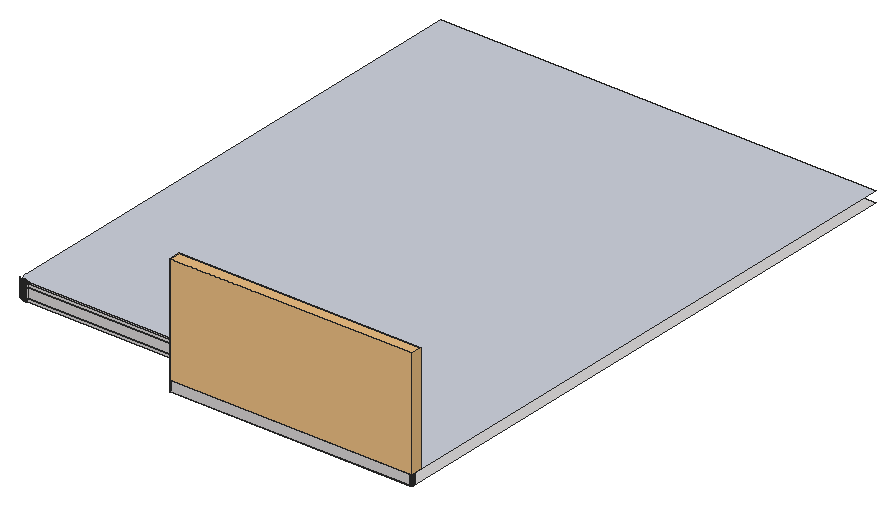
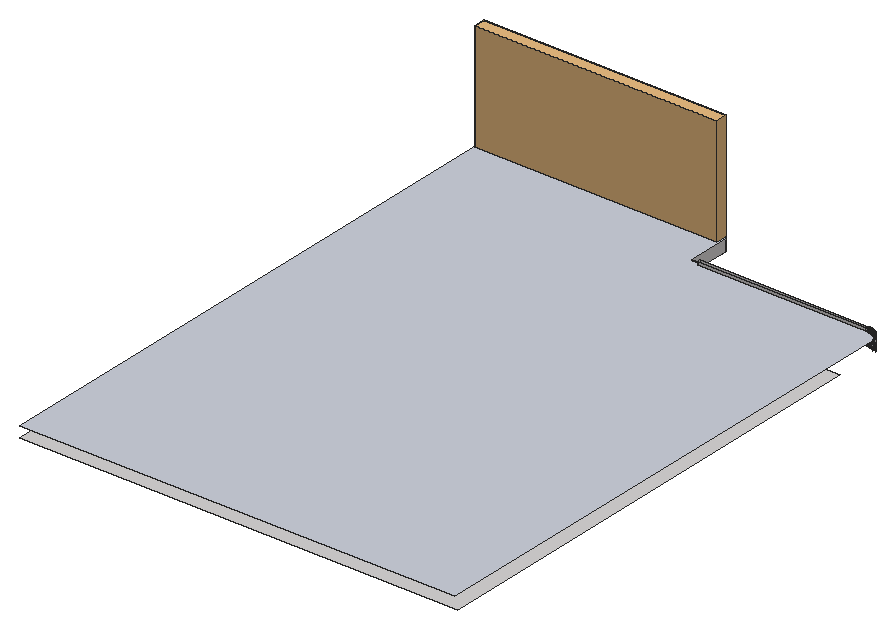
# SketchUp Ruby script. Lengths in inches.
U = 1.inch
M = Sketchup.active_model
def pt(a) = Geom::Point3d.new(a.map { |v| v * U })
def face(e, loops, mat)
  f = e.add_face(loops[0].map { |a| pt(a) })
  loops[1..].each { |l| e.add_face(l.map { |a| pt(a) }).erase! }
  f.material = f.back_material = mat if mat
  f
end
# faces: each face lists its corners as indices into pts; further lists are holes
def faces(e, pts, list, mat = nil) = list.each { |f| face(e, (f[0].is_a?(Array) ? f : [f]).map { |l| l.map { |i| pts[i] } }, mat) }
# xy, xz, yz: faces in a plane at the given z, y or x. An outline is a flat list of corners, or four numbers for a rectangle; further outlines are holes
def ring(l) = l.size == 4 ? [[l[0], l[1]], [l[2], l[1]], [l[2], l[3]], [l[0], l[3]]] : l.each_slice(2).to_a
def flat(e, list, mat, &to3) = list.each { |f| face(e, (f[0].is_a?(Array) ? f : [f]).map { |l| ring(l).map { |u, v| to3.(u, v) } }, mat) }
def xy(e, z, list, mat = nil) = flat(e, list, mat) { |x, y| [x, y, z] }
def xz(e, y, list, mat = nil) = flat(e, list, mat) { |x, z| [x, y, z] }
def yz(e, x, list, mat = nil) = flat(e, list, mat) { |y, z| [x, y, z] }
def lines(e, pts, list) = list.each { |a, b| e.add_line(pt(pts[a]), pt(pts[b])) }
# prism: a flat outline (further loops are holes) pulled along v
def prism(e, loops, v, mat = nil)
  f = face(e, loops, mat); d = Geom::Vector3d.new(v.map { |x| x * U })
  f.pushpull(f.normal.samedirection?(d) ? d.length : -d.length)
end
def box(e, o, s, mat = nil) = prism(e, [[o, [o[0] + s[0], o[1], o[2]], [o[0] + s[0], o[1] + s[1], o[2]], [o[0], o[1] + s[1], o[2]]]], [0, 0, s[2]], mat)
def at(x, y, z, deg = 0) = Geom::Transformation.translation(pt([x, y, z])) * Geom::Transformation.rotation(ORIGIN, Z_AXIS, deg.degrees)
def axes(o, x, y, z) = Geom::Transformation.new([*x, 0, *y, 0, *z, 0, *pt(o).to_a, 1])
def part(name) = M.definitions.add(name)
# library, detail: a bought-in or finely detailed component or shape, given as its bounding box
def library(name, o, s) = part(name).tap { |d| box(d.entities, o, s) }
def detail(e, o, s) = box(e.add_group.entities, o, s)
def put(e, d, t, mat = nil) = e.add_instance(d, t).tap { |i| i.material = mat if mat }
def group(e, t, mat = nil) = e.add_group.tap { |g| g.transformation = t; g.material = mat if mat }.entities
root = M.entities
M.materials.add("[Marble Carrara Floor Tile]").color = [204, 208, 219]
M.materials.add("[Quartz Light Brown]").color = [215, 212, 212]
c1 = library("Garniza_zaclona",[1.52,0,0],[127.96,8.15,78.72])
xy(root,246,[[215.88,155,215.76,155.01,215.65,155.02,215.41,155.06,215.3,155.08,215.1875,155.11,215.07,155.15,214.96,155.1875,214.85,155.23,214.74,155.28,214.64,155.33,214.53,155.38,214.43,155.44,214.33,155.51,214.24,155.57,214.14,155.64,213.96,155.8,213.8,155.96,213.64,156.14,213.57,156.24,213.51,156.33,213.44,156.43,213.38,156.53,213.33,156.64,213.28,156.74,213.23,156.85,213.15,157.07,213.11,157.1875,213.08,157.3,213.06,157.42,213.04,157.53,213.02,157.65,213.01,157.76,213,157.88,213,205,204,205,204,266,0,266,0,794,483,794,483,157.88,482.99,157.76,482.98,157.65,482.96,157.53,482.94,157.42,482.92,157.3,482.89,157.1875,482.85,157.07,482.8125,156.96,482.77,156.85,482.72,156.74,482.67,156.64,482.62,156.53,482.56,156.43,482.49,156.33,482.43,156.24,482.36,156.14,482.2,155.96,482.04,155.8,481.86,155.64,481.76,155.57,481.67,155.51,481.57,155.44,481.47,155.38,481.36,155.33,481.26,155.28,481.15,155.23,481.04,155.1875,480.93,155.15,480.8125,155.11,480.7,155.08,480.59,155.06,480.35,155.02,480.24,155.01,480.12,155]],"[Quartz Light Brown]")
xy(root,258,[[215.88,155,480.12,155,480.24,155.01,480.35,155.02,480.59,155.06,480.7,155.08,480.8125,155.11,480.93,155.15,481.04,155.1875,481.15,155.23,481.26,155.28,481.36,155.33,481.47,155.38,481.57,155.44,481.67,155.51,481.76,155.57,481.86,155.64,482.04,155.8,482.2,155.96,482.36,156.14,482.43,156.24,482.49,156.33,482.56,156.43,482.62,156.53,482.67,156.64,482.72,156.74,482.77,156.85,482.8125,156.96,482.85,157.07,482.89,157.1875,482.92,157.3,482.94,157.42,482.96,157.53,482.98,157.65,482.99,157.76,483,157.88,483,794,3,794,3,222.8,3.01,222.61,3.01,222.41,3.02,222.21,3.03,222.02,3.05,221.82,3.0625,221.63,3.08,221.43,3.1,221.24,3.13,221.04,3.16,220.85,3.18,220.65,3.22,220.46,3.25,220.27,3.29,220.07,3.41,219.5,3.51,219.12,3.5625,218.93,3.62,218.74,3.67,218.55,3.73,218.36,3.8,218.18,3.86,217.99,3.93,217.81,4.07,217.44,4.14,217.26,4.46,216.54,4.55,216.37,4.63,216.19,4.73,216.02,4.82,215.84,4.91,215.67,5.21,215.16,5.3125,215,5.42,214.83,5.53,214.67,5.64,214.5,5.86,214.18,5.98,214.03,6.22,213.71,6.34,213.56,6.47,213.41,6.59,213.26,6.85,212.96,6.99,212.82,7.12,212.67,7.26,212.53,7.39,212.39,7.53,212.26,7.67,212.12,7.82,211.99,7.96,211.85,8.26,211.59,8.41,211.47,8.56,211.34,8.71,211.22,9.03,210.98,9.18,210.86,9.5,210.64,9.67,210.53,9.83,210.42,10,210.3125,10.16,210.21,10.67,209.91,10.84,209.82,11.02,209.73,11.19,209.63,11.37,209.55,11.54,209.46,12.26,209.14,12.44,209.07,12.81,208.93,12.99,208.86,13.18,208.8,13.36,208.73,13.55,208.67,13.74,208.62,13.93,208.5625,14.12,208.51,14.5,208.41,15.07,208.29,15.27,208.25,15.46,208.22,15.65,208.18,15.85,208.16,16.04,208.13,16.24,208.1,16.43,208.08,16.63,208.0625,16.82,208.05,17.02,208.03,17.21,208.02,17.41,208.01,17.61,208.01,17.8,208,204,208,204,205,213,205,213,157.88,213.01,157.76,213.02,157.65,213.04,157.53,213.06,157.42,213.08,157.3,213.11,157.1875,213.15,157.07,213.23,156.85,213.28,156.74,213.33,156.64,213.38,156.53,213.44,156.43,213.51,156.33,213.57,156.24,213.64,156.14,213.8,155.96,213.96,155.8,214.14,155.64,214.24,155.57,214.33,155.51,214.43,155.44,214.53,155.38,214.64,155.33,214.74,155.28,214.85,155.23,214.96,155.1875,215.07,155.15,215.1875,155.11,215.3,155.08,215.41,155.06,215.65,155.02,215.76,155.01]],"[Marble Carrara Floor Tile]")
xz(root,155,[[215.88,246,216,258],[216,246,480,258],[480,246,480.12,258]],"[Quartz Light Brown]")
xz(root,205,[[17.76,243,18,246],[18,243,204,246],[204,246,213,246,213,258,204,258,204,257,18,257,18,247,204,247],[17.76,247,18,257],[17.76,258,18,261],
  [18,258,204,261]],"[Quartz Light Brown]")
xz(root,205.01,[[17.29,243,17.53,246],[17.29,247,17.53,257],[17.29,258,17.53,261]],"[Quartz Light Brown]")
xz(root,205.5,[[17.77,246,18,247],[18,246,204,247],[17.77,257,18,258],[18,257,204,258]],"[Quartz Light Brown]")
xz(root,205.51,[[17.3125,246,17.54,247],[17.3125,257,17.54,258]],"[Quartz Light Brown]")
xz(root,207,[[17.79,243,18,249],[18,243,202,249]],"[Quartz Light Brown]")
xz(root,207.01,[[17.37,243,17.58,249]],"[Quartz Light Brown]")
xz(root,208,[[17.8,258,18,261],[18,258,204,261]],"[Quartz Light Brown]")
xz(root,208.01,[[17.41,258,17.61,261]],"[Quartz Light Brown]")
yz(root,204,[[205,246,205.5,247],[205,257,205.5,258],[205,258,208,261]],"[Quartz Light Brown]")
yz(root,213,[[157.88,246,158,258],[158,246,205,258]],"[Quartz Light Brown]")
yz(root,483,[[157.88,246,158,258]],"[Quartz Light Brown]")
p = [[16.59,205.06,246],[16.59,205.06,243],[16.82,205.04,243],[16.82,205.04,246],[17.06,205.02,243],[17.06,205.02,246],
  [17.29,205.01,243],[17.29,205.01,246],[17.53,205.01,246],[17.53,205.01,243],[17.76,205,243],[17.76,205,246],
  [15.65,205.15,246],[15.65,205.15,243],[15.88,205.125,243],[15.88,205.125,246],[16.12,205.1,243],[16.12,205.1,246],
  [16.35,205.08,243],[16.35,205.08,246],[14.95,205.26,246],[14.95,205.26,243],[15.18,205.22,243],[15.18,205.22,246],
  [15.42,205.1875,243],[15.42,205.1875,246],[14.26,205.39,246],[14.26,205.39,243],[14.49,205.35,243],[14.49,205.35,246],
  [14.72,205.3,243],[14.72,205.3,246],[13.8,205.5,246],[13.8,205.5,243],[14.03,205.44,243],[14.03,205.44,246],
  [13.57,205.55,246],[13.57,205.55,243],[13.11,205.68,246],[13.11,205.68,243],[13.34,205.61,243],[13.34,205.61,246],
  [12.66,205.81,246],[12.66,205.81,243],[12.89,205.74,243],[12.89,205.74,246],[12.4375,205.88,246],[12.4375,205.88,243],
  [12.21,205.96,246],[12.21,205.96,243],[11.77,206.11,246],[11.77,206.11,243],[11.99,206.03,243],[11.99,206.03,246],
  [11.55,206.2,246],[11.55,206.2,243],[11.33,206.28,246],[11.33,206.28,243],[11.11,206.37,246],[11.11,206.37,243],
  [10.89,206.46,246],[10.89,206.46,243],[10.68,206.56,246],[10.68,206.56,243],[10.46,206.65,246],[10.46,206.65,243],
  [10.25,206.75,246],[10.25,206.75,243],[10.04,206.86,246],[10.04,206.86,243],[9.83,206.96,246],[9.83,206.96,243],
  [9.62,207.07,246],[9.62,207.07,243],[16.54,207.07,249],[16.74,207.05,249],[16.74,207.05,243],[16.54,207.07,243],
  [16.95,207.03,249],[16.95,207.03,243],[17.16,207.02,249],[17.16,207.02,243],[17.37,207.01,249],[17.37,207.01,243],
  [17.58,207.01,249],[17.79,207,249],[17.79,207,243],[17.58,207.01,243],[9.41,207.18,246],[9.41,207.18,243],
  [15.7,207.17,249],[15.91,207.14,249],[15.91,207.14,243],[15.7,207.17,243],[16.12,207.11,249],[16.12,207.11,243],
  [16.33,207.09,249],[16.33,207.09,243],[9.2,207.3,246],[9.2,207.3,243],[15.08,207.27,249],[15.29,207.23,249],
  [15.29,207.23,243],[15.08,207.27,243],[15.5,207.2,249],[15.5,207.2,243],[9,207.41,246],[9,207.41,243],
  [14.47,207.39,249],[14.67,207.35,249],[14.67,207.35,243],[14.47,207.39,243],[14.88,207.31,249],[14.88,207.31,243],
  [8.8,207.53,246],[8.8,207.53,243],[14.0625,207.49,249],[14.26,207.44,249],[14.26,207.44,243],[14.0625,207.49,243],
  [8.6,207.65,246],[8.6,207.65,243],[13.66,207.6,249],[13.86,207.55,249],[13.86,207.55,243],[13.66,207.6,243],
  [13.46,207.66,249],[13.46,207.66,243],[8.39,207.78,246],[8.39,207.78,243],[13.06,207.78,249],[13.26,207.72,249],
  [13.26,207.72,243],[13.06,207.78,243],[8.2,207.9,246],[8.2,207.9,243],[12.66,207.92,249],[12.86,207.85,249],
  [12.86,207.85,243],[12.66,207.92,243],[8,208.03,246],[8,208.03,243],[12.46,207.99,249],[12.46,207.99,243],
  [7.8,208.17,246],[7.8,208.17,243],[12.27,208.0625,249],[12.27,208.0625,243],[11.88,208.22,249],[12.07,208.14,249],
  [12.07,208.14,243],[11.88,208.22,243],[7.61,208.3,246],[7.61,208.3,243],[11.68,208.3,249],[11.68,208.3,243],
  [7.42,208.4375,246],[7.42,208.4375,243],[11.49,208.38,249],[11.49,208.38,243],[7.23,208.58,246],[7.23,208.58,243],
  [11.3,208.47,249],[11.3,208.47,243],[11.11,208.56,249],[11.11,208.56,243],[7.04,208.72,246],[7.04,208.72,243],
  [10.92,208.65,249],[10.92,208.65,243],[6.86,208.86,246],[6.86,208.86,243],[10.55,208.84,249],[10.74,208.74,249],
  [10.74,208.74,243],[10.55,208.84,243],[10.37,208.9375,249],[10.37,208.9375,243],[6.67,209.01,246],[6.67,209.01,243],
  [10.18,209.04,249],[10.18,209.04,243],[6.49,209.16,246],[6.49,209.16,243],[10,209.14,249],[10,209.14,243],
  [9.82,209.25,249],[9.82,209.25,243],[6.31,209.3125,246],[6.31,209.3125,243],[9.64,209.36,249],[9.64,209.36,243],
  [6.13,209.47,246],[6.13,209.47,243],[9.46,209.47,249],[9.46,209.47,243],[5.96,209.625,246],[5.96,209.625,243],
  [9.29,209.58,249],[9.29,209.58,243],[5.78,209.78,246],[5.78,209.78,243],[9.11,209.7,249],[9.11,209.7,243],
  [8.9375,209.8125,249],[8.9375,209.8125,243],[5.61,209.94,246],[5.61,209.94,243],[8.77,209.93,249],[8.77,209.93,243],
  [5.44,210.11,246],[5.44,210.11,243],[8.6,210.06,249],[8.6,210.06,243],[5.27,210.27,246],[5.27,210.27,243],
  [8.43,210.18,249],[8.43,210.18,243],[8.26,210.31,249],[8.26,210.31,243],[215.53,155.04,258],[215.41,155.06,258],
  [215.41,155.06,246],[215.53,155.04,246],[215.65,155.02,258],[215.65,155.02,246],[215.76,155.01,258],[215.76,155.01,246],
  [215.88,155,258],[215.88,155,246],[480.24,155.01,258],[480.12,155,258],[480.12,155,246],[480.24,155.01,246],
  [480.35,155.02,258],[480.35,155.02,246],[480.47,155.04,258],[480.47,155.04,246],[480.59,155.06,258],[480.59,155.06,246],
  [215.07,155.15,258],[214.96,155.1875,258],[214.96,155.1875,246],[215.07,155.15,246],[215.1875,155.11,258],[215.1875,155.11,246],
  [215.3,155.08,258],[215.3,155.08,246],[480.7,155.08,258],[480.7,155.08,246],[480.8125,155.11,258],[480.8125,155.11,246],
  [480.93,155.15,258],[480.93,155.15,246],[481.04,155.1875,258],[481.04,155.1875,246],[214.85,155.23,258],[214.74,155.28,258],
  [214.74,155.28,246],[214.85,155.23,246],[481.15,155.23,258],[481.15,155.23,246],[481.26,155.28,258],[481.26,155.28,246],
  [214.64,155.33,258],[214.53,155.38,258],[214.53,155.38,246],[214.64,155.33,246],[481.36,155.33,258],[481.36,155.33,246],
  [481.47,155.38,258],[481.47,155.38,246],[214.43,155.44,258],[214.33,155.51,258],[214.33,155.51,246],[214.43,155.44,246],
  [481.57,155.44,258],[481.57,155.44,246],[481.67,155.51,258],[481.67,155.51,246],[214.24,155.57,258],[214.24,155.57,246],
  [481.76,155.57,258],[481.76,155.57,246],[214.14,155.64,258],[214.14,155.64,246],[214.05,155.72,258],[214.05,155.72,246],
  [481.86,155.64,258],[481.86,155.64,246],[481.95,155.72,258],[481.95,155.72,246],[213.96,155.8,258],[213.96,155.8,246],
  [482.04,155.8,258],[482.04,155.8,246],[213.88,155.88,258],[213.88,155.88,246],[482.12,155.88,258],[482.12,155.88,246],
  [213.8,155.96,258],[213.8,155.96,246],[482.2,155.96,258],[482.2,155.96,246],[213.72,156.05,258],[213.72,156.05,246],
  [482.28,156.05,258],[482.28,156.05,246],[213.64,156.14,258],[213.64,156.14,246],[213.57,156.24,258],[213.57,156.24,246],
  [482.36,156.14,258],[482.36,156.14,246],[482.43,156.24,258],[482.43,156.24,246],[213.51,156.33,258],[213.51,156.33,246],
  [482.49,156.33,258],[482.49,156.33,246],[213.44,156.43,258],[213.44,156.43,246],[482.56,156.43,258],[482.56,156.43,246],
  [213.38,156.53,258],[213.38,156.53,246],[482.62,156.53,258],[482.62,156.53,246],[213.33,156.64,258],[213.33,156.64,246],
  [482.67,156.64,258],[482.67,156.64,246],[213.28,156.74,258],[213.28,156.74,246],[482.72,156.74,258],[482.72,156.74,246],
  [213.23,156.85,258],[213.23,156.85,246],[482.77,156.85,258],[482.77,156.85,246],[213.19,156.96,258],[213.19,156.96,246],
  [482.8125,156.96,258],[482.8125,156.96,246],[213.15,157.07,258],[213.15,157.07,246],[482.85,157.07,258],[482.85,157.07,246],
  [213.11,157.1875,258],[213.11,157.1875,246],[482.89,157.1875,258],[482.89,157.1875,246],[213.08,157.3,258],[213.08,157.3,246],
  [482.92,157.3,258],[482.92,157.3,246],[213.06,157.42,258],[213.06,157.42,246],[482.94,157.42,258],[482.94,157.42,246],
  [213.04,157.53,258],[213.04,157.53,246],[482.96,157.53,258],[482.96,157.53,246],[213.02,157.65,258],[213.02,157.65,246],
  [482.98,157.65,258],[482.98,157.65,246],[213.01,157.76,258],[213.01,157.76,246],[482.99,157.76,258],[482.99,157.76,246],
  [213,157.88,258],[213,157.88,246],[483,157.88,258],[483,157.88,246],[16.625,205.55,247],[16.625,205.55,246],
  [16.86,205.54,246],[16.86,205.54,247],[17.08,205.52,246],[17.08,205.52,247],[17.3125,205.51,246],[17.3125,205.51,247],
  [17.54,205.51,247],[17.54,205.51,246],[17.77,205.5,246],[17.77,205.5,247],[15.49,205.68,247],[15.49,205.68,246],
  [15.72,205.65,246],[15.72,205.65,247],[15.94,205.62,246],[15.94,205.62,247],[16.17,205.6,246],[16.17,205.6,247],
  [16.4,205.57,246],[16.4,205.57,247],[15.04,205.75,247],[15.04,205.75,246],[15.26,205.72,246],[15.26,205.72,247],
  [14.36,205.88,247],[14.36,205.88,246],[14.59,205.84,246],[14.59,205.84,247],[14.8125,205.79,246],[14.8125,205.79,247],
  [13.91,205.98,247],[13.91,205.98,246],[14.14,205.93,246],[14.14,205.93,247],[13.47,206.1,247],[13.47,206.1,246],
  [13.69,206.04,246],[13.69,206.04,247],[13.25,206.16,247],[13.25,206.16,246],[12.8125,206.29,247],[12.8125,206.29,246],
  [13.03,206.22,246],[13.03,206.22,247],[12.59,206.36,247],[12.59,206.36,246],[12.16,206.5,247],[12.16,206.5,246],
  [12.375,206.43,246],[12.375,206.43,247],[11.94,206.58,247],[11.94,206.58,246],[11.73,206.66,247],[11.73,206.66,246],
  [11.3,206.83,247],[11.3,206.83,246],[11.52,206.75,246],[11.52,206.75,247],[11.09,206.92,247],[11.09,206.92,246],
  [10.88,207.01,247],[10.88,207.01,246],[10.67,207.11,247],[10.67,207.11,246],[10.47,207.2,247],[10.47,207.2,246],
  [10.26,207.3,247],[10.26,207.3,246],[10.06,207.41,247],[10.06,207.41,246],[9.85,207.51,247],[9.85,207.51,246],
  [9.65,207.62,247],[9.65,207.62,246],[9.45,207.73,247],[9.45,207.73,246],[9.25,207.84,247],[9.25,207.84,246],
  [9.05,207.96,247],[9.05,207.96,246],[8.86,208.08,247],[8.86,208.08,246],[8.66,208.2,247],[8.66,208.2,246],
  [8.47,208.32,247],[8.47,208.32,246],[8.28,208.45,247],[8.28,208.45,246],[8.09,208.58,247],[8.09,208.58,246],
  [7.9,208.71,247],[7.9,208.71,246],[7.71,208.84,247],[7.71,208.84,246],[7.53,208.98,247],[7.53,208.98,246],
  [7.35,209.12,247],[7.35,209.12,246],[7.17,209.26,247],[7.17,209.26,246],[6.99,209.4,247],[6.99,209.4,246],
  [6.81,209.55,247],[6.81,209.55,246],[6.63,209.69,247],[6.63,209.69,246],[6.46,209.84,247],[6.46,209.84,246],
  [6.29,209.99,247],[6.29,209.99,246],[6.12,210.15,247],[6.12,210.15,246],[5.95,210.31,247],[5.95,210.31,246],
  [16.59,205.06,257],[16.59,205.06,247],[16.82,205.04,247],[16.82,205.04,257],[17.06,205.02,247],[17.06,205.02,257],
  [17.29,205.01,247],[17.29,205.01,257],[17.53,205.01,257],[17.53,205.01,247],[17.76,205,247],[17.76,205,257],
  [15.65,205.15,257],[15.65,205.15,247],[15.88,205.125,247],[15.88,205.125,257],[16.12,205.1,247],[16.12,205.1,257],
  [16.35,205.08,247],[16.35,205.08,257],[14.95,205.26,257],[14.95,205.26,247],[15.18,205.22,247],[15.18,205.22,257],
  [15.42,205.1875,247],[15.42,205.1875,257],[14.26,205.39,257],[14.26,205.39,247],[14.49,205.35,247],[14.49,205.35,257],
  [14.72,205.3,247],[14.72,205.3,257],[13.8,205.5,257],[13.8,205.5,247],[14.03,205.44,247],[14.03,205.44,257],
  [13.57,205.55,257],[13.57,205.55,247],[13.11,205.68,257],[13.11,205.68,247],[13.34,205.61,247],[13.34,205.61,257],
  [12.66,205.81,257],[12.66,205.81,247],[12.89,205.74,247],[12.89,205.74,257],[12.4375,205.88,257],[12.4375,205.88,247],
  [12.21,205.96,257],[12.21,205.96,247],[11.77,206.11,257],[11.77,206.11,247],[11.99,206.03,247],[11.99,206.03,257],
  [11.55,206.2,257],[11.55,206.2,247],[11.33,206.28,257],[11.33,206.28,247],[11.11,206.37,257],[11.11,206.37,247],
  [10.89,206.46,257],[10.89,206.46,247],[10.68,206.56,257],[10.68,206.56,247],[10.46,206.65,257],[10.46,206.65,247],
  [10.25,206.75,257],[10.25,206.75,247],[10.04,206.86,257],[10.04,206.86,247],[9.83,206.96,257],[9.83,206.96,247],
  [9.62,207.07,257],[9.62,207.07,247],[9.41,207.18,257],[9.41,207.18,247],[9.2,207.3,257],[9.2,207.3,247],
  [9,207.41,257],[9,207.41,247],[8.8,207.53,257],[8.8,207.53,247],[8.6,207.65,257],[8.6,207.65,247],
  [8.39,207.78,257],[8.39,207.78,247],[8.2,207.9,257],[8.2,207.9,247],[8,208.03,257],[8,208.03,247],
  [7.8,208.17,257],[7.8,208.17,247],[7.61,208.3,257],[7.61,208.3,247],[7.42,208.4375,257],[7.42,208.4375,247],
  [7.23,208.58,257],[7.23,208.58,247],[7.04,208.72,257],[7.04,208.72,247],[6.86,208.86,257],[6.86,208.86,247],
  [6.67,209.01,257],[6.67,209.01,247],[6.49,209.16,257],[6.49,209.16,247],[6.31,209.3125,257],[6.31,209.3125,247],
  [6.13,209.47,257],[6.13,209.47,247],[5.96,209.625,257],[5.96,209.625,247],[5.78,209.78,257],[5.78,209.78,247],
  [5.61,209.94,257],[5.61,209.94,247],[5.44,210.11,257],[5.44,210.11,247],[5.27,210.27,257],[5.27,210.27,247],
  [16.625,205.55,258],[16.625,205.55,257],[16.86,205.54,257],[16.86,205.54,258],[17.08,205.52,257],[17.08,205.52,258],
  [17.3125,205.51,257],[17.3125,205.51,258],[17.54,205.51,258],[17.54,205.51,257],[17.77,205.5,257],[17.77,205.5,258],
  [15.49,205.68,258],[15.49,205.68,257],[15.72,205.65,257],[15.72,205.65,258],[15.94,205.62,257],[15.94,205.62,258],
  [16.17,205.6,257],[16.17,205.6,258],[16.4,205.57,257],[16.4,205.57,258],[15.04,205.75,258],[15.04,205.75,257],
  [15.26,205.72,257],[15.26,205.72,258],[14.36,205.88,258],[14.36,205.88,257],[14.59,205.84,257],[14.59,205.84,258],
  [14.8125,205.79,257],[14.8125,205.79,258],[13.91,205.98,258],[13.91,205.98,257],[14.14,205.93,257],[14.14,205.93,258],
  [13.47,206.1,258],[13.47,206.1,257],[13.69,206.04,257],[13.69,206.04,258],[13.25,206.16,258],[13.25,206.16,257],
  [12.8125,206.29,258],[12.8125,206.29,257],[13.03,206.22,257],[13.03,206.22,258],[12.59,206.36,258],[12.59,206.36,257],
  [12.16,206.5,258],[12.16,206.5,257],[12.375,206.43,257],[12.375,206.43,258],[11.94,206.58,258],[11.94,206.58,257],
  [11.73,206.66,258],[11.73,206.66,257],[11.3,206.83,258],[11.3,206.83,257],[11.52,206.75,257],[11.52,206.75,258],
  [11.09,206.92,258],[11.09,206.92,257],[10.88,207.01,258],[10.88,207.01,257],[10.67,207.11,258],[10.67,207.11,257],
  [10.47,207.2,258],[10.47,207.2,257],[10.26,207.3,258],[10.26,207.3,257],[10.06,207.41,258],[10.06,207.41,257],
  [9.85,207.51,258],[9.85,207.51,257],[9.65,207.62,258],[9.65,207.62,257],[9.45,207.73,258],[9.45,207.73,257],
  [9.25,207.84,258],[9.25,207.84,257],[9.05,207.96,258],[9.05,207.96,257],[8.86,208.08,258],[8.86,208.08,257],
  [8.66,208.2,258],[8.66,208.2,257],[8.47,208.32,258],[8.47,208.32,257],[8.28,208.45,258],[8.28,208.45,257],
  [8.09,208.58,258],[8.09,208.58,257],[7.9,208.71,258],[7.9,208.71,257],[7.71,208.84,258],[7.71,208.84,257],
  [7.53,208.98,258],[7.53,208.98,257],[7.35,209.12,258],[7.35,209.12,257],[7.17,209.26,258],[7.17,209.26,257],
  [6.99,209.4,258],[6.99,209.4,257],[6.81,209.55,258],[6.81,209.55,257],[6.63,209.69,258],[6.63,209.69,257],
  [6.46,209.84,258],[6.46,209.84,257],[6.29,209.99,258],[6.29,209.99,257],[6.12,210.15,258],[6.12,210.15,257],
  [5.95,210.31,258],[5.95,210.31,257],[16.82,205.04,258],[16.82,205.04,261],[16.59,205.06,261],[16.59,205.06,258],
  [17.06,205.02,258],[17.06,205.02,261],[17.29,205.01,258],[17.29,205.01,261],[17.76,205,258],[17.76,205,261],
  [17.53,205.01,261],[17.53,205.01,258],[15.88,205.125,258],[15.88,205.125,261],[15.65,205.15,261],[15.65,205.15,258],
  [16.12,205.1,258],[16.12,205.1,261],[16.35,205.08,258],[16.35,205.08,261],[15.18,205.22,258],[15.18,205.22,261],
  [14.95,205.26,261],[14.95,205.26,258],[15.42,205.1875,258],[15.42,205.1875,261],[14.49,205.35,258],[14.49,205.35,261],
  [14.26,205.39,261],[14.26,205.39,258],[14.72,205.3,258],[14.72,205.3,261],[14.03,205.44,258],[14.03,205.44,261],
  [13.8,205.5,261],[13.8,205.5,258],[13.57,205.55,261],[13.57,205.55,258],[13.34,205.61,258],[13.34,205.61,261],
  [13.11,205.68,261],[13.11,205.68,258],[12.89,205.74,258],[12.89,205.74,261],[12.66,205.81,261],[12.66,205.81,258],
  [12.4375,205.88,261],[12.4375,205.88,258],[12.21,205.96,261],[12.21,205.96,258],[11.99,206.03,258],[11.99,206.03,261],
  [11.77,206.11,261],[11.77,206.11,258],[11.55,206.2,261],[11.55,206.2,258],[11.33,206.28,261],[11.33,206.28,258],
  [11.11,206.37,261],[11.11,206.37,258],[10.89,206.46,261],[10.89,206.46,258],[10.68,206.56,261],[10.68,206.56,258],
  [10.46,206.65,261],[10.46,206.65,258],[10.25,206.75,261],[10.25,206.75,258],[10.04,206.86,261],[10.04,206.86,258],
  [9.83,206.96,261],[9.83,206.96,258],[9.62,207.07,261],[9.62,207.07,258],[9.41,207.18,261],[9.41,207.18,258],
  [9.2,207.3,261],[9.2,207.3,258],[9,207.41,261],[9,207.41,258],[8.8,207.53,261],[8.8,207.53,258],
  [8.6,207.65,261],[8.6,207.65,258],[8.39,207.78,261],[8.39,207.78,258],[8.2,207.9,261],[8.2,207.9,258],
  [8,208.03,261],[8,208.03,258],[7.8,208.17,261],[7.8,208.17,258],[16.82,208.05,258],[16.63,208.0625,258],
  [16.63,208.0625,261],[16.82,208.05,261],[17.02,208.03,258],[17.02,208.03,261],[17.21,208.02,258],[17.21,208.02,261],
  [17.41,208.01,258],[17.41,208.01,261],[17.8,208,258],[17.61,208.01,258],[17.61,208.01,261],[17.8,208,261],
  [16.04,208.13,258],[15.85,208.16,258],[15.85,208.16,261],[16.04,208.13,261],[16.24,208.1,258],[16.24,208.1,261],
  [16.43,208.08,258],[16.43,208.08,261],[7.61,208.3,261],[7.61,208.3,258],[15.46,208.22,258],[15.27,208.25,258],
  [15.27,208.25,261],[15.46,208.22,261],[15.65,208.18,258],[15.65,208.18,261],[7.42,208.4375,261],[7.42,208.4375,258],
  [14.88,208.33,258],[14.69,208.37,258],[14.69,208.37,261],[14.88,208.33,261],[15.07,208.29,258],[15.07,208.29,261],
  [7.23,208.58,261],[7.23,208.58,258],[14.5,208.41,258],[14.31,208.46,258],[14.31,208.46,261],[14.5,208.41,261],
  [14.12,208.51,258],[13.93,208.5625,258],[13.93,208.5625,261],[14.12,208.51,261],[7.04,208.72,261],[7.04,208.72,258],
  [13.74,208.62,258],[13.55,208.67,258],[13.55,208.67,261],[13.74,208.62,261],[6.86,208.86,261],[6.86,208.86,258],
  [13.36,208.73,258],[13.18,208.8,258],[13.18,208.8,261],[13.36,208.73,261],[12.99,208.86,258],[12.99,208.86,261],
  [6.67,209.01,261],[6.67,209.01,258],[12.81,208.93,258],[12.625,209,258],[12.625,209,261],[12.81,208.93,261],
  [6.49,209.16,261],[6.49,209.16,258],[12.44,209.07,258],[12.44,209.07,261],[12.26,209.14,258],[12.08,209.22,258],
  [12.08,209.22,261],[12.26,209.14,261],[6.31,209.3125,261],[6.31,209.3125,258],[11.9,209.3,258],[11.9,209.3,261],
  [6.13,209.47,261],[6.13,209.47,258],[11.72,209.38,258],[11.72,209.38,261],[11.54,209.46,258],[11.54,209.46,261],
  [5.96,209.625,261],[5.96,209.625,258],[11.37,209.55,258],[11.19,209.63,258],[11.19,209.63,261],[11.37,209.55,261],
  [5.78,209.78,261],[5.78,209.78,258],[11.02,209.73,258],[11.02,209.73,261],[10.84,209.82,258],[10.84,209.82,261],
  [5.61,209.94,261],[5.61,209.94,258],[10.67,209.91,258],[10.67,209.91,261],[5.44,210.11,261],[5.44,210.11,258],
  [10.5,210.01,258],[10.5,210.01,261],[10.33,210.11,258],[10.33,210.11,261],[5.27,210.27,261],[5.27,210.27,258],
  [10.16,210.21,258],[10.16,210.21,261],[10,210.3125,258],[10,210.3125,261]]
faces(root,p,[[0,1,2,3],[3,2,4,5],[5,4,6,7],[8,9,10,11],[12,13,14,15],[15,14,16,17],[17,16,18,19],[19,18,1,0],
  [20,21,22,23],[23,22,24,25],[25,24,13,12],[26,27,28,29],[29,28,30,31],[31,30,21,20],[32,33,34,35],[35,34,27,26],
  [36,37,33,32],[38,39,40,41],[41,40,37,36],[42,43,44,45],[45,44,39,38],[46,47,43,42],[48,49,47,46],[50,51,52,53],
  [53,52,49,48],[54,55,51,50],[56,57,55,54],[58,59,57,56],[60,61,59,58],[62,63,61,60],[64,65,63,62],[66,67,65,64],
  [68,69,67,66],[70,71,69,68],[72,73,71,70],[74,75,76,77],[75,78,79,76],[78,80,81,79],[80,82,83,81],[84,85,86,87],
  [88,89,73,72],[90,91,92,93],[91,94,95,92],[94,96,97,95],[96,74,77,97],[98,99,89,88],[100,101,102,103],[101,104,105,102],
  [104,90,93,105],[106,107,99,98],[108,109,110,111],[109,112,113,110],[112,100,103,113],[114,115,107,106],[116,117,118,119],[117,108,111,118],
  [120,121,115,114],[122,123,124,125],[123,116,119,124],[126,122,125,127],[128,129,121,120],[130,131,132,133],[131,126,127,132],[134,135,129,128],
  [136,137,138,139],[137,130,133,138],[140,141,135,134],[142,136,139,143],[144,145,141,140],[146,142,143,147],[148,149,150,151],[149,146,147,150],
  [152,153,145,144],[154,148,151,155],[156,157,153,152],[158,154,155,159],[160,161,157,156],[162,158,159,163],[164,162,163,165],[166,167,161,160],
  [168,164,165,169],[170,171,167,166],[172,173,174,175],[173,168,169,174],[176,172,175,177],[178,179,171,170],[180,176,177,181],[182,183,179,178],
  [184,180,181,185],[186,184,185,187],[188,189,183,182],[190,186,187,191],[192,193,189,188],[194,190,191,195],[196,197,193,192],[198,194,195,199],
  [200,201,197,196],[202,198,199,203],[204,202,203,205],[206,207,201,200],[208,204,205,209],[210,211,207,206],[212,208,209,213],[214,215,211,210],
  [216,212,213,217],[218,216,217,219],[220,221,222,223],[224,220,223,225],[226,224,225,227],[228,226,227,229],[230,231,232,233],[234,230,233,235],
  [236,234,235,237],[238,236,237,239],[240,241,242,243],[244,240,243,245],[246,244,245,247],[221,246,247,222],[248,238,239,249],[250,248,249,251],
  [252,250,251,253],[254,252,253,255],[256,257,258,259],[241,256,259,242],[260,254,255,261],[262,260,261,263],[264,265,266,267],[257,264,267,258],
  [268,262,263,269],[270,268,269,271],[272,273,274,275],[265,272,275,266],[276,270,271,277],[278,276,277,279],[273,280,281,274],[282,278,279,283],
  [280,284,285,281],[284,286,287,285],[288,282,283,289],[290,288,289,291],[286,292,293,287],[294,290,291,295],[292,296,297,293],[298,294,295,299],
  [296,300,301,297],[302,298,299,303],[300,304,305,301],[306,302,303,307],[304,308,309,305],[308,310,311,309],[312,306,307,313],[314,312,313,315],
  [310,316,317,311],[318,314,315,319],[316,320,321,317],[322,318,319,323],[320,324,325,321],[326,322,323,327],[324,328,329,325],[330,326,327,331],
  [328,332,333,329],[334,330,331,335],[332,336,337,333],[338,334,335,339],[336,340,341,337],[342,338,339,343],[340,344,345,341],[346,342,343,347],
  [344,348,349,345],[350,346,347,351],[348,352,353,349],[354,350,351,355],[352,356,357,353],[358,354,355,359],[356,360,361,357],[362,358,359,363],
  [360,364,365,361],[366,362,363,367],[364,368,369,365],[370,366,367,371],[368,372,373,369],[374,370,371,375],[376,377,378,379],[379,378,380,381],
  [381,380,382,383],[384,385,386,387],[388,389,390,391],[391,390,392,393],[393,392,394,395],[395,394,396,397],[397,396,377,376],[398,399,400,401],
  [401,400,389,388],[402,403,404,405],[405,404,406,407],[407,406,399,398],[408,409,410,411],[411,410,403,402],[412,413,414,415],[415,414,409,408],
  [416,417,413,412],[418,419,420,421],[421,420,417,416],[422,423,419,418],[424,425,426,427],[427,426,423,422],[428,429,425,424],[430,431,429,428],
  [432,433,434,435],[435,434,431,430],[436,437,433,432],[438,439,437,436],[440,441,439,438],[442,443,441,440],[444,445,443,442],[446,447,445,444],
  [448,449,447,446],[450,451,449,448],[452,453,451,450],[454,455,453,452],[456,457,455,454],[458,459,457,456],[460,461,459,458],[462,463,461,460],
  [464,465,463,462],[466,467,465,464],[468,469,467,466],[470,471,469,468],[472,473,471,470],[474,475,473,472],[476,477,475,474],[478,479,477,476],
  [480,481,479,478],[482,483,481,480],[484,485,483,482],[486,487,485,484],[488,489,487,486],[490,491,489,488],[492,493,494,495],[495,494,496,497],
  [497,496,498,499],[500,501,502,503],[504,505,506,507],[507,506,508,509],[509,508,510,511],[511,510,493,492],[512,513,514,515],[515,514,516,517],
  [517,516,505,504],[518,519,520,521],[521,520,522,523],[523,522,513,512],[524,525,526,527],[527,526,519,518],[528,529,525,524],[530,531,532,533],
  [533,532,529,528],[534,535,536,537],[537,536,531,530],[538,539,535,534],[540,541,539,538],[542,543,544,545],[545,544,541,540],[546,547,543,542],
  [548,549,547,546],[550,551,549,548],[552,553,551,550],[554,555,553,552],[556,557,555,554],[558,559,557,556],[560,561,559,558],[562,563,561,560],
  [564,565,563,562],[566,567,565,564],[568,569,567,566],[570,571,569,568],[572,573,571,570],[574,575,573,572],[576,577,575,574],[578,579,577,576],
  [580,581,579,578],[582,583,581,580],[584,585,583,582],[586,587,585,584],[588,589,587,586],[590,591,589,588],[592,593,591,590],[594,595,593,592],
  [596,597,595,594],[598,599,597,596],[600,601,599,598],[602,603,601,600],[604,605,603,602],[606,607,605,604],[608,609,607,606],[610,611,609,608],
  [612,613,614,615],[615,614,616,617],[617,616,618,619],[620,621,622,623],[624,625,626,627],[627,626,628,629],[629,628,630,631],[631,630,632,633],
  [633,632,613,612],[634,635,636,637],[637,636,625,624],[638,639,640,641],[641,640,642,643],[643,642,635,634],[644,645,646,647],[647,646,639,638],
  [648,649,650,651],[651,650,645,644],[652,653,649,648],[654,655,656,657],[657,656,653,652],[658,659,655,654],[660,661,662,663],[663,662,659,658],
  [664,665,661,660],[666,667,665,664],[668,669,670,671],[671,670,667,666],[672,673,669,668],[674,675,673,672],[676,677,675,674],[678,679,677,676],
  [680,681,679,678],[682,683,681,680],[684,685,683,682],[686,687,685,684],[688,689,687,686],[690,691,689,688],[692,693,691,690],[694,695,693,692],
  [696,697,695,694],[698,699,697,696],[700,701,699,698],[702,703,701,700],[704,705,703,702],[706,707,705,704],[708,709,707,706],[710,711,709,708],
  [712,713,711,710],[714,715,713,712],[716,717,715,714],[718,719,717,716],[720,721,719,718],[722,723,721,720],[724,725,723,722],[726,727,725,724],
  [728,729,730,731],[732,733,729,728],[734,735,733,732],[736,737,738,739],[740,741,742,743],[744,745,741,740],[746,747,745,744],[731,730,747,746],
  [748,749,750,751],[752,753,749,748],[743,742,753,752],[754,755,756,757],[758,759,755,754],[751,750,759,758],[760,761,762,763],[757,756,761,760],
  [763,762,764,765],[766,767,768,769],[765,764,767,766],[770,771,772,773],[769,768,771,770],[773,772,774,775],[775,774,776,777],[778,779,780,781],
  [777,776,779,778],[781,780,782,783],[783,782,784,785],[785,784,786,787],[787,786,788,789],[789,788,790,791],[791,790,792,793],[793,792,794,795],
  [795,794,796,797],[797,796,798,799],[799,798,800,801],[801,800,802,803],[803,802,804,805],[805,804,806,807],[807,806,808,809],[809,808,810,811],
  [811,810,812,813],[813,812,814,815],[815,814,816,817],[817,816,818,819],[820,821,822,823],[824,820,823,825],[826,824,825,827],[828,826,827,829],
  [830,831,832,833],[834,835,836,837],[838,834,837,839],[840,838,839,841],[821,840,841,822],[819,818,842,843],[844,845,846,847],[848,844,847,849],
  [835,848,849,836],[843,842,850,851],[852,853,854,855],[856,852,855,857],[845,856,857,846],[851,850,858,859],[860,861,862,863],[853,860,863,854],
  [864,865,866,867],[861,864,867,862],[859,858,868,869],[870,871,872,873],[865,870,873,866],[869,868,874,875],[876,877,878,879],[871,876,879,872],
  [877,880,881,878],[875,874,882,883],[884,885,886,887],[880,884,887,881],[883,882,888,889],[885,890,891,886],[892,893,894,895],[890,892,895,891],
  [889,888,896,897],[893,898,899,894],[897,896,900,901],[898,902,903,899],[902,904,905,903],[901,900,906,907],[908,909,910,911],[904,908,911,905],
  [907,906,912,913],[909,914,915,910],[914,916,917,915],[913,912,918,919],[916,920,921,917],[919,918,922,923],[920,924,925,921],[924,926,927,925],
  [923,922,928,929],[926,930,931,927],[930,932,933,931]],"[Quartz Light Brown]")
put(root,c1,axes([213,154.04,258],[2.08532,0,0],[0,1.49,0],[0,0,1.52445]))
